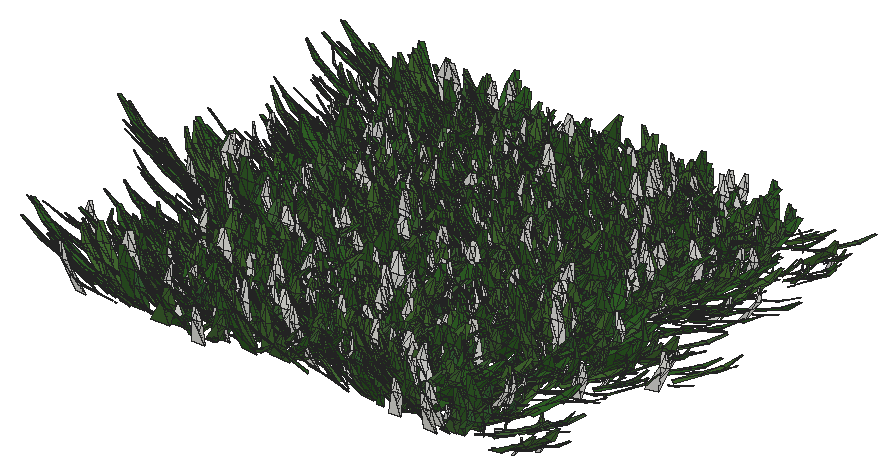
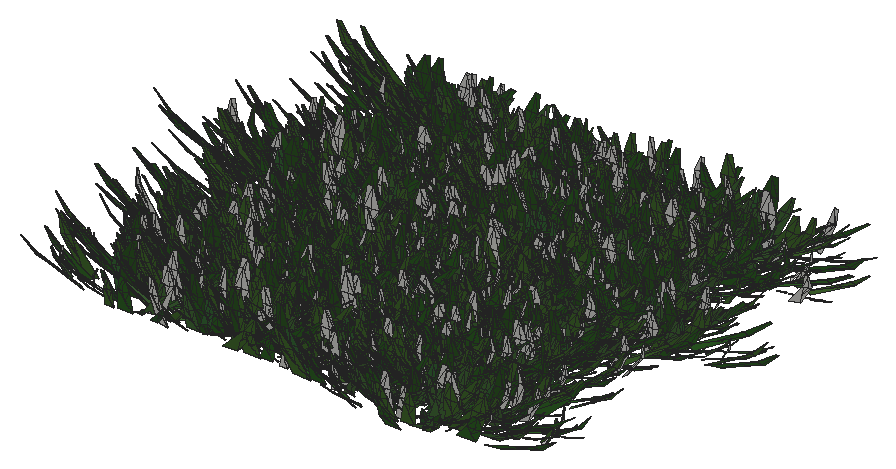
# SketchUp Ruby script. Lengths in inches.
U = 1.inch
M = Sketchup.active_model
def pt(a) = Geom::Point3d.new(a.map { |v| v * U })
def face(e, loops, mat)
  f = e.add_face(loops[0].map { |a| pt(a) })
  loops[1..].each { |l| e.add_face(l.map { |a| pt(a) }).erase! }
  f.material = f.back_material = mat if mat
  f
end
# faces: each face lists its corners as indices into pts; further lists are holes
def faces(e, pts, list, mat = nil) = list.each { |f| face(e, (f[0].is_a?(Array) ? f : [f]).map { |l| l.map { |i| pts[i] } }, mat) }
# xy, xz, yz: faces in a plane at the given z, y or x. An outline is a flat list of corners, or four numbers for a rectangle; further outlines are holes
def ring(l) = l.size == 4 ? [[l[0], l[1]], [l[2], l[1]], [l[2], l[3]], [l[0], l[3]]] : l.each_slice(2).to_a
def flat(e, list, mat, &to3) = list.each { |f| face(e, (f[0].is_a?(Array) ? f : [f]).map { |l| ring(l).map { |u, v| to3.(u, v) } }, mat) }
def xy(e, z, list, mat = nil) = flat(e, list, mat) { |x, y| [x, y, z] }
def xz(e, y, list, mat = nil) = flat(e, list, mat) { |x, z| [x, y, z] }
def yz(e, x, list, mat = nil) = flat(e, list, mat) { |y, z| [x, y, z] }
def lines(e, pts, list) = list.each { |a, b| e.add_line(pt(pts[a]), pt(pts[b])) }
# prism: a flat outline (further loops are holes) pulled along v
def prism(e, loops, v, mat = nil)
  f = face(e, loops, mat); d = Geom::Vector3d.new(v.map { |x| x * U })
  f.pushpull(f.normal.samedirection?(d) ? d.length : -d.length)
end
def box(e, o, s, mat = nil) = prism(e, [[o, [o[0] + s[0], o[1], o[2]], [o[0] + s[0], o[1] + s[1], o[2]], [o[0], o[1] + s[1], o[2]]]], [0, 0, s[2]], mat)
def at(x, y, z, deg = 0) = Geom::Transformation.translation(pt([x, y, z])) * Geom::Transformation.rotation(ORIGIN, Z_AXIS, deg.degrees)
def axes(o, x, y, z) = Geom::Transformation.new([*x, 0, *y, 0, *z, 0, *pt(o).to_a, 1])
def part(name) = M.definitions.add(name)
# library, detail: a bought-in or finely detailed component or shape, given as its bounding box
def library(name, o, s) = part(name).tap { |d| box(d.entities, o, s) }
def detail(e, o, s) = box(e.add_group.entities, o, s)
def put(e, d, t, mat = nil) = e.add_instance(d, t).tap { |i| i.material = mat if mat }
def group(e, t, mat = nil) = e.add_group.tap { |g| g.transformation = t; g.material = mat if mat }.entities
root = M.entities
M.materials.add("Material10").color = [48, 100, 38]
M.materials.add("Material3").color = [68, 110, 58]
M.materials.add("Material4").color = [48, 90, 38]
M.materials.add("Material5").color = [68, 110, 48]
M.materials.add("Material6").color = [48, 90, 48]
M.materials.add("Material7").color = [58, 110, 58]
M.materials.add("Material8").color = [58, 90, 38]
M.materials.add("Material9").color = [68, 100, 58]
c1 = part("grass00")
p = [[-0.6875,0.15,0],[-0.56,0.08,5.52],[-0.04,0.03,2.76],[0.48,-0.02,0],[0.35,-0.02,5.52],[-0.1,-0.14,5.52],
  [-0.12,0.65,8.37],[-0.42,0.65,8.37]]
faces(c1.entities,p,[[0,1,2,3],[3,2,4],[1,5,2],[5,4,2],[1,6,5],[4,5,6],[7,6,1]])
c2 = part("Group16\#1")
put(c2.entities,c1,axes([1.44,-0.61,-0.01],[0.05352,0.12609,0],[-0.10704,0.04543,0.07239],[0.06664,-0.02828,0.11628]),"Material6")
put(c2.entities,c1,axes([0.76,-0.15,-0.01],[0.04676,0.24062,0],[-0.23162,0.04501,0.06642],[0.0652,-0.01267,0.23595]),"Material3")
put(c2.entities,c1,axes([0.79,0.01,-0.01],[-0.00606,0.34651,0],[-0.34381,-0.00602,0.0432],[0.04319,0.00076,0.34386]))
put(c2.entities,c1,axes([1,0.23,-0.01],[-0.07192,0.31144,0],[-0.28722,-0.06632,0.1236],[0.12043,0.02781,0.29478]),"Material5")
put(c2.entities,c1,axes([1.66,0.77,-0.01],[-0.13828,0.29651,0],[-0.21551,-0.1005,0.22471],[0.20365,0.09498,0.23779]),"Material10")
put(c2.entities,c1,axes([0.6875,0.52,-0.01],[-0.18126,0.24051,0],[-0.22746,-0.17142,0.09788],[0.07817,0.05891,0.28481]),"Material5")
put(c2.entities,c1,axes([0.68,0.78,-0.01],[-0.215,0.18688,0],[-0.12385,-0.14248,0.21334],[0.13995,0.16101,0.18878]),"Material3")
put(c2.entities,c1,axes([0.56,1,-0.01],[-0.13756,0.07624,0],[-0.06159,-0.11112,0.0927],[0.04494,0.08108,0.12705]),"Material5")
put(c2.entities,c1,axes([0.2,0.64,-0.01],[-0.23729,0.07254,0],[-0.05711,-0.18681,0.153],[0.04473,0.14632,0.19535]),"Material10")
put(c2.entities,c1,axes([0.0625,0.72,-0.01],[-0.28874,0.02525,0],[-0.02179,-0.24916,0.14647],[0.01276,0.14591,0.25012]),"Material3")
put(c2.entities,c1,axes([-0.08,0.62,-0.01],[-0.34089,-0.04187,0],[0.03255,-0.26504,0.216],[-0.02633,0.21439,0.26703]),"Material10")
put(c2.entities,c1,axes([-0.34,0.98,-0.01],[-0.14314,-0.0493,0],[0.04397,-0.12769,0.06843],[-0.02228,0.0647,0.13505]),"Material10")
put(c2.entities,c1,axes([-0.87,1.45,-0.01],[-0.23488,-0.14114,0],[0.13761,-0.22901,0.06087],[-0.03135,0.05217,0.26717]))
put(c2.entities,c1,axes([-0.72,0.77,-0.01],[-0.14208,-0.13251,0],[0.07209,-0.0773,0.16301],[-0.11118,0.11922,0.1057]),"Material10")
put(c2.entities,c1,axes([-0.62,0.43,-0.01],[-0.14845,-0.21203,0],[0.18654,-0.13061,0.12304],[-0.10079,0.07057,0.22772]),"Material3")
put(c2.entities,c1,axes([-0.68,0.29,-0.01],[-0.13639,-0.32136,0],[0.31723,-0.13464,0.05579],[-0.05136,0.0218,0.34462]),"Material4")
put(c2.entities,c1,axes([-0.64,0.125,-0.01],[-0.0458,-0.23569,0],[0.22124,-0.043,0.08276],[-0.08124,0.01579,0.22538]),"Material7")
put(c2.entities,c1,axes([-1.6,-0.03,-0.01],[0.00576,-0.32897,0],[0.27526,0.00482,0.18018],[-0.18015,-0.00315,0.2753]),"Material5")
put(c2.entities,c1,axes([-1.36,-0.31,-0.01],[0.05718,-0.24765,0],[0.18172,0.04196,0.17267],[-0.16825,-0.03885,0.1865]),"Material10")
put(c2.entities,c1,axes([-1.54,-0.72,-0.01],[0.06537,-0.14017,0],[0.13555,0.06321,0.03939],[-0.0357,-0.01665,0.14956]))
put(c2.entities,c1,axes([-1.19,-0.9,-0.01],[0.09597,-0.12735,0],[0.11214,0.08451,0.07557],[-0.06035,-0.04548,0.14042]),"Material9")
put(c2.entities,c1,axes([-0.47,-0.54,-0.01],[0.11588,-0.10072,0],[0.0618,0.0711,0.12124],[-0.07953,-0.0915,0.0942]))
put(c2.entities,c1,axes([-0.47,-0.84,-0.01],[0.11927,-0.0661,0],[0.06603,0.11913,0.00646],[-0.00313,-0.00565,0.13621]),"Material5")
put(c2.entities,c1,axes([-0.38,-1.24,-0.01],[0.28037,-0.08571,0],[0.0618,0.20215,0.20315],[-0.05939,-0.19428,0.21139]),"Material9")
put(c2.entities,c1,axes([-0.06,-0.66,-0.01],[0.22719,-0.01987,0],[0.01247,0.14255,0.17758],[-0.01547,-0.17691,0.1431]),"Material8")
put(c2.entities,c1,axes([0.11,-0.89,-0.01],[0.14882,0.01828,0],[-0.01058,0.08611,0.12229],[0.01491,-0.12138,0.08676]),"Material6")
put(c2.entities,c1,axes([0.25,-0.72,-0.01],[0.20481,0.07053,0],[-0.06206,0.18022,0.10291],[0.03351,-0.0973,0.1906]),"Material6")
put(c2.entities,c1,axes([0.85,-1.42,-0.01],[0.16481,0.09904,0],[-0.09472,0.15762,0.05616],[0.02893,-0.04814,0.18389]),"Material5")
put(c2.entities,c1,axes([1.01,-1.09,-0.01],[0.21858,0.20385,0],[-0.17495,0.1876,0.15339],[0.10462,-0.11218,0.25652]),"Material10")
put(c2.entities,c1,axes([1.01,-0.71,-0.01],[0.08733,0.12473,0],[-0.06445,0.04512,0.13037],[0.1068,-0.07477,0.07867]),"Material6")
c3 = part("Group15\#1")
put(c3.entities,c2,at(0,0,0))
c4 = part("3darcstudiotree_grass00\#1")
put(c4.entities,c3,at(0,0,0))
put(root,c4,axes([921.625,950.11,0],[-2.89172,1.0734,0],[-3.89316,-0.6555,-0.0002],[-0.00109,-0.00018,1.96126]))
put(root,c4,axes([922,951.05,0],[4.74483,-0.24076,0],[0.85247,1.04999,-0.04034],[0.05471,0.06739,1.82611]))
put(root,c4,axes([923.99,968.21,0],[-3.63628,-0.62096,0],[2.92947,-1.07217,-0.03279],[0.09663,-0.03537,1.69581]))
put(root,c4,axes([921.97,938.41,0],[4.00198,0.55005,0],[-2.10991,0.95943,-0.0244],[-0.05644,0.02566,1.31386]))
put(root,c4,axes([924.61,951.62,0],[-4.89778,-0.29998,0],[1.23144,-1.25658,-0.038],[0.05293,-0.05401,1.89315]))
put(root,c4,axes([924.41,933.5,0],[-1.90201,1.02558,0],[-4.52641,-0.52466,-0.04346],[-0.2357,-0.02732,1.86413]))
put(root,c4,axes([924.58,963.82,0],[3.74508,0.15378,0],[-0.63868,0.9721,-0.00501],[-0.00465,0.00708,1.40942]))
put(root,c4,axes([924.51,970.26,0],[0.68514,1.26478,0],[-4.89254,0.16565,-0.03426],[-0.19489,0.0066,1.77113]))
put(root,c4,axes([925.28,959.25,0],[3.3533,-0.38731,0],[1.56438,0.84651,-0.0238],[0.08194,0.04434,1.9133]))
put(root,c4,axes([925.79,947.01,0],[2.65179,-0.82671,0],[3.59664,0.72105,-0.04277],[0.18565,0.03722,1.60323]))
put(root,c4,axes([926.85,939.54,0],[-4.93357,-0.09351,0],[0.37181,-1.22601,-0.05601],[0.01916,-0.06319,1.39118]))
put(root,c4,axes([926.99,942.43,0],[-3.34759,-0.83293,0],[3.286,-0.82541,-0.05331],[0.22185,-0.05573,1.71744]))
put(root,c4,axes([926.98,940.55,0],[0.64604,-1.03899,0],[4.47986,0.1741,-0.01704],[0.10727,0.00417,1.80481]))
put(root,c4,axes([925.39,937.53,0],[1.02925,1.26191,0],[-4.50486,0.22964,-0.03996],[-0.19294,0.00984,1.416]))
put(root,c4,axes([925.4,957.25,0],[2.0369,1.16411,0],[-3.53478,0.38656,-0.02724],[-0.15553,0.01701,1.50258]))
put(root,c4,axes([925.71,945.89,0],[4.16551,0.00829,0],[-0.03133,0.98341,-0.01492],[-0.00089,0.02794,1.84219]))
put(root,c4,axes([925.75,935.03,0],[3.29102,0.44295,0],[-1.77478,0.82413,-0.02125],[-0.05688,0.02641,1.32121]))
put(root,c4,axes([926.7,970.76,0],[-2.38266,1.15159,0],[-4.35256,-0.56285,-0.04288],[-0.20993,-0.02715,1.68813]))
put(root,c4,axes([926.88,952.92,0],[-2.09957,0.91209,0],[-4.41964,-0.63586,-0.03664],[-0.13193,-0.01898,1.3241]))
put(root,c4,axes([926.61,962.3125,0],[3.03097,0.54961,0],[-2.11734,0.72979,-0.02439],[-0.10216,0.03521,1.60766]))
put(root,c4,axes([927.14,948.41,0],[4.80677,-0.31921,0],[1.29296,1.21686,-0.06211],[0.08115,0.07638,1.60192]))
put(root,c4,axes([927.98,965.28,0],[1.96449,-0.88015,0],[3.48703,0.48644,-0.05199],[0.25829,0.03603,1.41973]))
put(root,c4,axes([927.64,960.8,0],[-2.15894,0.75531,0],[-3.65102,-0.65224,-0.01309],[-0.05957,-0.01064,1.56859]))
put(root,c4,axes([926.875,967.23,0],[3.46841,0.85303,0],[-2.60309,0.66151,-0.00671],[-0.03109,0.0079,1.53359]))
put(root,c4,axes([926.85,956.64,0],[4.28051,0.69294,0],[-2.55654,0.98703,-0.02279],[-0.07934,0.03063,1.88252]))
put(root,c4,axes([927.48,949.89,0],[4.57656,0.58892,0],[-2.21831,1.07741,-0.04224],[-0.10111,0.04911,1.58426]))
put(root,c4,axes([927.93,935.85,0],[3.90944,0.05539,0],[-0.24036,1.06035,-0.02759],[-0.00929,0.04097,1.57942]))
put(root,c4,axes([927.84,972.53,0],[1.41495,1.18383,0],[-3.49756,0.26127,-0.01522],[-0.0888,0.00663,1.38916]))
put(root,c4,axes([929.91,944.99,0],[-4.73179,-0.12886,0],[0.46967,-1.07792,-0.0047],[0.00279,-0.0064,1.4854]))
put(root,c4,axes([928.2,954.96,0],[0.18591,1.26274,0],[-5.04075,0.04638,-0.03073],[-0.14495,0.00133,1.48809]))
put(root,c4,axes([929.98,964.77,0],[-4.30621,-0.01829,0],[0.08217,-1.20899,-0.03595],[0.00336,-0.04947,1.66434]))
put(root,c4,axes([930.31,956.45,0],[-3.87854,-0.40989,0],[1.77421,-1.04926,-0.0473],[0.09277,-0.05486,1.43445]))
put(root,c4,axes([928.33,944.15,0],[4.45359,0.5299,0],[-1.68792,0.88663,-0.01473],[-0.03849,0.02022,1.49308]))
put(root,c4,axes([930.07,947.27,0],[-4.3672,0.54864,0],[-1.80768,-0.89932,-0.0516],[-0.17927,-0.08919,1.94674]))
put(root,c4,axes([930.65,950,0],[-4.20222,0.09704,0],[-0.34915,-0.94494,-0.04806],[-0.02957,-0.08003,1.58689]))
put(root,c4,axes([930.38,963.16,0],[2.2244,-0.73123,0],[4.08618,0.77689,-0.04371],[0.15259,0.02901,1.40723]))
put(root,c4,axes([930.62,933.21,0],[-3.5275,0.23131,0],[-1.26087,-1.2018,-0.03948],[-0.051,-0.04861,1.58152]))
put(root,c4,axes([931.44,969.78,0],[-4.09129,-0.53085,0],[1.96428,-0.94617,-0.02416],[0.06052,-0.02915,1.4491]))
put(root,c4,axes([931.49,968.04,0],[-3.27232,-0.38033,0],[1.61038,-0.86597,-0.04575],[0.12951,-0.06964,1.60296]))
put(root,c4,axes([930.3,959.49,0],[1.34498,0.85271,0],[-3.61197,0.35607,-0.04901],[-0.30956,0.03052,1.64754]))
put(root,c4,axes([931.5625,941.91,0],[-3.74465,0.10964,0],[-0.44388,-0.94751,-0.03745],[-0.02749,-0.05868,1.50509]))
put(root,c4,axes([930.15,937.94,0],[0.55868,1.18187,0],[-4.38906,0.12967,-0.00527],[-0.02848,0.00084,1.50433]))
put(root,c4,axes([930.8,971.66,0],[3.92571,-0.06568,0],[0.27031,1.00981,-0.02393],[0.00951,0.03553,1.50627]))
put(root,c4,axes([930.66,957.33,0],[4.1204,0.14772,0],[-0.55424,0.96623,-0.02285],[-0.01788,0.03117,1.34478]))
put(root,c4,axes([932.27,934.97,0],[-4.54837,0.61423,0],[-2.27056,-1.05085,-0.03525],[-0.07342,-0.03398,1.3087]))
put(root,c4,axes([932.45,939.78,0],[1.35556,-1.09662,0],[3.48641,0.26935,-0.00928],[0.07297,0.00564,1.87692]))
put(root,c4,axes([931.18,948.62,0],[4.58081,0.57203,0],[-2.05118,1.02662,-0.04234],[-0.09467,0.04738,1.4356]))
put(root,c4,axes([931.75,962.35,0],[4.09069,0.39107,0],[-1.49345,0.97637,-0.02441],[-0.06576,0.04299,1.97124]))
put(root,c4,axes([931.72,960.57,0],[4.67312,0.46375,0],[-1.55175,0.97728,-0.04113],[-0.07938,0.05,1.37498]))
put(root,c4,axes([932.28,966.34,0],[1.74991,0.88126,0],[-3.81182,0.47307,-0.01001],[-0.04959,0.00615,1.4706]))
put(root,c4,axes([934.3,954.01,0],[-4.64971,-0.14285,0],[0.57946,-1.17887,-0.04768],[0.02933,-0.05967,1.49744]))
put(root,c4,axes([932.68,943.76,0],[0.96395,1.06005,0],[-4.81113,0.27344,-0.06457],[-0.29518,0.01678,1.44574]))
put(root,c4,axes([933.8,936.25,0],[3.00205,-0.85659,0],[3.63036,0.7952,-0.04981],[0.2075,0.04545,1.67091]))
put(root,c4,axes([932.82,952.7,0],[3.43592,0.73211,0],[-2.51322,0.73719,-0.00613],[-0.02752,0.00807,1.67562]))
put(root,c4,axes([933.76,940.36,0],[1.74385,0.8383,0],[-3.77239,0.49046,-0.03549],[-0.18091,0.02352,1.52707]))
put(root,c4,axes([933.53,951.63,0],[1.69559,1.05532,0],[-4.4836,0.45024,-0.00669],[-0.03988,0.004,1.94122]))
put(root,c4,axes([936.78,934.31,0],[-2.1334,-0.73078,0],[3.43772,-0.62725,-0.00015],[0.00089,-0.00016,1.94435]))
put(root,c4,axes([936.46,951.25,0],[-0.05318,-0.92593,0],[5.00241,-0.01796,-0.06189],[0.33029,-0.00119,1.66883]))
put(root,c4,axes([936.82,970.07,0],[-3.23712,-0.63399,0],[2.66966,-0.85194,-0.04081],[0.13619,-0.04346,1.46417]))
put(root,c4,axes([936.76,963.4,0],[-4.03858,-0.16836,0],[0.61274,-0.91864,-0.01602],[0.01597,-0.02395,1.41148]))
put(root,c4,axes([937.43,971.4,0],[-0.4686,-0.94109,0],[4.875,-0.15171,-0.05859],[0.34766,-0.01082,1.83593]))
put(root,c4,axes([937.8,956.05,0],[-4.976,0.12548,0],[-0.39366,-0.97566,-0.00469],[-0.00376,-0.00932,1.96044]))
put(root,c4,axes([938.07,957.69,0],[-3.93213,0.25374,0],[-1.01516,-0.98322,-0.03018],[-0.05893,-0.05707,1.98332]))
put(root,c4,axes([938.63,967.68,0],[-3.81287,-0.39073,0],[1.76767,-1.0781,-0.01809],[0.03493,-0.0213,1.4829]))
put(root,c4,axes([938.05,966.3125,0],[1.16902,-1.01976,0],[4.12301,0.2954,-0.03571],[0.25113,0.01799,1.9611]))
put(root,c4,axes([938.18,936.51,0],[-3.57612,0.46,0],[-1.68045,-0.8165,-0.01759],[-0.06739,-0.03274,1.92222]))
put(root,c4,axes([937.94,945.24,0],[2.75353,-0.91552,0],[4.13951,0.77813,-0.05965],[0.29097,0.05469,1.97549]))
put(root,c4,axes([937.08,960.57,0],[4.41787,0.20597,0],[-0.82473,1.10563,-0.00417],[-0.0051,0.00683,1.87295]))
put(root,c4,axes([938.8,946.4375,0],[-0.77256,-1.09422,0],[3.72876,-0.16454,-0.01992],[0.13289,-0.00586,1.60321]))
put(root,c4,axes([937.08,942.34,0],[4.90123,0.13236,0],[-0.55386,1.28181,-0.03307],[-0.01756,0.04064,1.59331]))
put(root,c4,axes([937.55,953.11,0],[0.63816,1.22279,0],[-3.70201,0.12075,-0.03746],[-0.26805,0.00874,1.68385]))
put(root,c4,axes([938.3,940.41,0],[-3.38877,0.51557,0],[-2.38455,-0.97958,-0.01391],[-0.04361,-0.01791,1.7292]))
put(root,c4,axes([938.53,943.57,0],[2.69835,-0.96968,0],[3.12111,0.54282,-0.02795],[0.17981,0.03127,1.86246]))
put(root,c4,axes([938.17,959.05,0],[-2.15572,1.01928,0],[-4.46043,-0.5896,-0.01892],[-0.07769,-0.01027,1.46501]))
put(root,c4,axes([940.08,965.1,0],[-3.178,-0.72198,0],[3.25819,-0.89636,-0.02206],[0.07961,-0.0219,1.62457]))
put(root,c4,axes([938.42,948.78,0],[-2.01821,1.07087,0],[-4.04462,-0.47641,-0.00165],[-0.00796,-0.00094,1.48801]))
put(root,c4,axes([940.17,937.46,0],[-5.04293,-0.12413,0],[0.46059,-1.16949,-0.00134],[0.0006,-0.00152,1.33719]))
put(root,c4,axes([938.11,962.59,0],[1.81913,1.13072,0],[-4.24624,0.42697,-0.0015],[-0.00751,0.00076,1.54039]))
put(root,c4,axes([939.71,939.39,0],[2.93485,-0.98597,0],[3.93521,0.7321,-0.05496],[0.20354,0.03787,1.41537]))
put(root,c4,axes([939.92,949.78,0],[0.69977,0.95429,0],[-4.68091,0.21453,-0.00804],[-0.04724,0.00217,1.77733]))
put(root,c4,axes([940.1875,954.9,0],[2.05265,1.08844,0],[-3.86298,0.45532,-0.03917],[-0.23834,0.02809,1.79585]))
put(root,c4,axes([942.94,937.68,0],[-1.12524,-0.96886,0],[3.74948,-0.27217,-0.00444],[0.03259,-0.00237,1.86591]))
put(root,c4,axes([942.3125,951.3,0],[1.4605,-0.95002,0],[3.8779,0.3726,-0.03841],[0.24153,0.02321,1.74904]))
put(root,c4,axes([942.83,957.26,0],[-2.14754,-0.73736,0],[3.76224,-0.68483,-0.06067],[0.30518,-0.05555,1.80988]))
put(root,c4,axes([942.71,940.76,0],[-3.33972,0.41247,0],[-1.92358,-0.97344,-0.03032],[-0.07425,-0.03758,1.50108]))
put(root,c4,axes([942.69,962.51,0],[3.71164,-0.61185,0],[2.58785,0.98115,-0.02666],[0.07433,0.02818,1.48784]))
put(root,c4,axes([943.79,971.05,0],[0.28174,-1.01382,0],[4.36389,0.07579,-0.0172],[0.10528,0.00183,1.67763]))
put(root,c4,axes([943.35,935.4,0],[-2.86097,0.86073,0],[-3.01972,-0.62732,-0.04997],[-0.22994,-0.04777,1.46822]))
put(root,c4,axes([944.54,961.15,0],[-4.12883,-0.65967,0],[2.58219,-1.01011,-0.05584],[0.19452,-0.07609,1.93872]))
put(root,c4,axes([943.05,939.77,0],[-0.2845,0.94758,0],[-4.0362,-0.07574,-0.02554],[-0.16533,-0.0031,1.64241]))
put(root,c4,axes([944.98,943.43,0],[-4.76231,0.21357,0],[-0.8747,-1.21904,-0.00093],[-0.00084,-0.00117,1.58752]))
put(root,c4,axes([943.68,936.63,0],[4.17112,0.04454,0],[-0.19892,1.16431,-0.01987],[-0.00428,0.02505,1.47043]))
put(root,c4,axes([943.71,945.35,0],[4.56851,-0.0546,0],[0.17436,0.91177,-0.03217],[0.01167,0.06102,1.73328]))
put(root,c4,axes([943.92,946.78,0],[4.23657,-0.2376,0],[0.80233,0.89415,-0.00297],[0.00478,0.00533,1.68702]))
put(root,c4,axes([945.77,968.15,0],[-3.12199,-0.46434,0],[2.64637,-1.11204,-0.00321],[0.00751,-0.00316,1.48019]))
put(root,c4,axes([944.91,963.2,0],[-3.87477,0.75183,0],[-2.84001,-0.9148,-0.03049],[-0.11215,-0.03613,1.73706]))
put(root,c4,axes([944.15,953.58,0],[3.58042,0.48605,0],[-1.82681,0.84106,-0.03457],[-0.13256,0.06103,1.92264]))
put(root,c4,axes([945.2,966.875,0],[2.19573,-0.79563,0],[3.28578,0.56674,-0.0362],[0.23043,0.03975,1.92943]))
put(root,c4,axes([944.77,942.7,0],[-1.60767,1.01804,0],[-4.53552,-0.44765,-0.02576],[-0.12044,-0.01189,1.53201]))
put(root,c4,axes([944.86,948.2,0],[4.66104,-0.01291,0],[0.04336,0.97863,-0.01976],[0.00122,0.02762,1.36845]))
put(root,c4,axes([945.11,955.97,0],[2.73136,0.67519,0],[-2.53096,0.63991,-0.02576],[-0.15171,0.03836,1.88472]))
put(root,c4,axes([945.22,958.6875,0],[4.8227,0.33397,0],[-1.37587,1.24178,-0.02222],[-0.03562,0.03215,1.93436]))
put(root,c4,axes([945.58,969.75,0],[2.66703,0.73786,0],[-3.13866,0.70905,-0.0306],[-0.16013,0.03617,1.86488]))
put(root,c4,axes([946.45,949.47,0],[-2.52556,0.85651,0],[-3.11909,-0.57482,-0.0238],[-0.1265,-0.02331,1.59896]))
put(root,c4,axes([945.74,965.6,0],[1.56451,1.00298,0],[-4.78607,0.4666,-0.01645],[-0.08409,0.0082,1.76201]))
put(root,c4,axes([946.04,955.06,0],[1.42494,0.93436,0],[-3.83119,0.36517,-0.01397],[-0.07753,0.00739,1.52193]))
put(root,c4,axes([948.24,933.39,0],[-3.93046,0.12235,0],[-0.4536,-0.91071,-0.03309],[-0.02864,-0.0575,1.60704]))
put(root,c4,axes([948.85,936.84,0],[-3.14311,-1.03345,0],[3.53925,-0.67276,-0.02],[0.10195,-0.01938,1.779]))
put(root,c4,axes([948.61,937.81,0],[-0.38253,-1.25706,0],[5.07372,-0.0965,-0.05882],[0.29497,-0.00561,1.5994]))
put(root,c4,axes([949.02,945.92,0],[-3.9211,-0.27648,0],[1.04934,-0.93013,-0.015],[0.02202,-0.01952,1.30652]))
put(root,c4,axes([948.14,968.35,0],[-0.95414,1.15068,0],[-4.04773,-0.20977,-0.02464],[-0.16776,-0.00869,1.79662]))
put(root,c4,axes([948.86,939.4,0],[-3.41535,0.94101,0],[-3.19182,-0.72403,-0.0082],[-0.03901,-0.00885,1.73071]))
put(root,c4,axes([948.55,967.05,0],[-0.26244,0.97433,0],[-4.33641,-0.073,-0.04305],[-0.28268,-0.00476,1.78778]))
put(root,c4,axes([949.7,955.55,0],[-4.734,0.44651,0],[-1.80443,-1.19569,-0.03096],[-0.06152,-0.04076,1.79846]))
put(root,c4,axes([950.3,944.38,0],[-3.54413,-0.35283,0],[1.88693,-1.18461,-0.01803],[0.03799,-0.02385,1.81493]))
put(root,c4,axes([949.12,952.85,0],[-1.93923,0.80033,0],[-4.36084,-0.6604,-0.05645],[-0.30002,-0.04543,1.97994]))
put(root,c4,axes([950.59,964.14,0],[-1.73824,-0.83269,0],[3.93121,-0.5129,-0.00435],[0.02089,-0.00273,1.50222]))
put(root,c4,axes([948.96,951.68,0],[3.26249,0.60372,0],[-2.60827,0.88094,-0.05487],[-0.17274,0.05834,1.44987]))
put(root,c4,axes([949.07,969.61,0],[0.73959,1.18717,0],[-3.65318,0.14224,-0.00889],[-0.05312,0.00207,1.39664]))
put(root,c4,axes([949.93,971.43,0],[2.83501,-0.87969,0],[3.07253,0.61887,-0.02709],[0.15503,0.03123,1.8123]))
put(root,c4,axes([948.96,960.89,0],[4.22317,0.50582,0],[-2.02967,1.05913,-0.04599],[-0.0924,0.04822,1.36526]))
put(root,c4,axes([951.21,964.85,0],[-3.49567,-0.41418,0],[1.84622,-0.97387,-0.03887],[0.09057,-0.04778,1.46596]))
put(root,c4,axes([950.3,950.18,0],[3.68446,-0.69974,0],[2.40562,0.79167,-0.03309],[0.11614,0.03822,1.44206]))
put(root,c4,axes([951.69,957.39,0],[-3.25249,-0.4237,0],[1.99269,-0.95605,-0.0201],[0.0448,-0.0215,1.30027]))
put(root,c4,axes([951.89,942.27,0],[-3.91695,-0.76183,0],[3.11851,-1.00211,-0.06227],[0.16525,-0.0531,1.37168]))
put(root,c4,axes([949.96,961.99,0],[1.52552,1.07764,0],[-3.72178,0.32929,-0.0171],[-0.12069,0.01068,1.84743]))
put(root,c4,axes([950.65,935.11,0],[-0.98833,1.19917,0],[-3.8776,-0.19974,-0.03296],[-0.18407,-0.00948,1.411]))
put(root,c4,axes([950.82,948.41,0],[-1.74933,1.03948,0],[-3.53507,-0.37182,-0.02216],[-0.14167,-0.0149,1.66252]))
put(root,c4,axes([951.95,958.61,0],[3.35043,-0.75633,0],[2.9183,0.80798,-0.04418],[0.18264,0.05057,1.67893]))
put(root,c4,axes([951.68,940.61,0],[-0.82221,1.07388,0],[-4.85232,-0.2322,-0.01652],[-0.07909,-0.00378,1.50529]))
put(root,c4,axes([951.89,954.49,0],[4.38567,-0.08429,0],[0.3564,1.15903,-0.03486],[0.01549,0.05039,1.68524]))
put(root,c4,axes([952.33,946.79,0],[4.19452,0.71588,0],[-2.43274,0.89088,-0.02215],[-0.08774,0.03213,1.8946]))
put(root,c4,axes([954.36,957.63,0],[0.50446,-1.28497,0],[4.75288,0.11662,-0.05803],[0.25331,0.00622,1.30918]))
put(root,c4,axes([955.23,960.77,0],[-3.01986,-0.89757,0],[3.46122,-0.72782,-0.04595],[0.21791,-0.04582,1.75181]))
put(root,c4,axes([954.71,962.6,0],[2.394,-0.81419,0],[3.9298,0.72218,-0.0227],[0.09655,0.01774,1.60931]))
put(root,c4,axes([954.77,933.33,0],[-3.78924,0.73867,0],[-2.26636,-0.72662,-0.02241],[-0.08836,-0.02833,1.47722]))
put(root,c4,axes([955.49,944.04,0],[-4.0317,-0.25141,0],[0.95302,-0.95517,-0.04204],[0.06722,-0.06737,1.62585]))
put(root,c4,axes([955.125,934.74,0],[-4.15536,0.77828,0],[-2.7986,-0.93389,-0.03017],[-0.1071,-0.03574,1.72726]))
put(root,c4,axes([954.34,959.38,0],[1.24349,0.95069,0],[-4.25943,0.34821,-0.05705],[-0.29582,0.02418,1.52794]))
put(root,c4,axes([956.19,967.25,0],[-3.8617,-0.01302,0],[0.05631,-1.04356,-0.03579],[0.00298,-0.05513,1.60809]))
put(root,c4,axes([955.52,951.54,0],[-3.40266,0.70782,0],[-3.16523,-0.95101,-0.01948],[-0.07283,-0.02188,1.80807]))
put(root,c4,axes([955.81,971.75,0],[-3.32672,0.63857,0],[-2.74378,-0.89337,-0.05552],[-0.19615,-0.06387,1.63365]))
put(root,c4,axes([954.56,964.68,0],[1.64031,0.90171,0],[-3.63622,0.41342,-0.00419],[-0.02649,0.00301,1.73548]))
put(root,c4,axes([955.76,949.8,0],[3.62794,-0.3827,0],[1.97795,1.17191,-0.0407],[0.07531,0.04462,1.51351]))
put(root,c4,axes([954.95,936.9,0],[3.52874,0.5715,0],[-2.37881,0.918,-0.01048],[-0.03241,0.01251,1.55517]))
put(root,c4,axes([957.3,948.63,0],[-4.67502,-0.56796,0],[2.06884,-1.06432,-0.01545],[0.04157,-0.02139,1.8215]))
put(root,c4,axes([954.96,967.88,0],[2.90908,1.00895,0],[-3.39125,0.61112,-0.01552],[-0.0694,0.01251,1.43977]))
put(root,c4,axes([955.89,945.41,0],[0.16489,0.91256,0],[-4.05383,0.04578,-0.0329],[-0.25692,0.0029,1.98251]))
